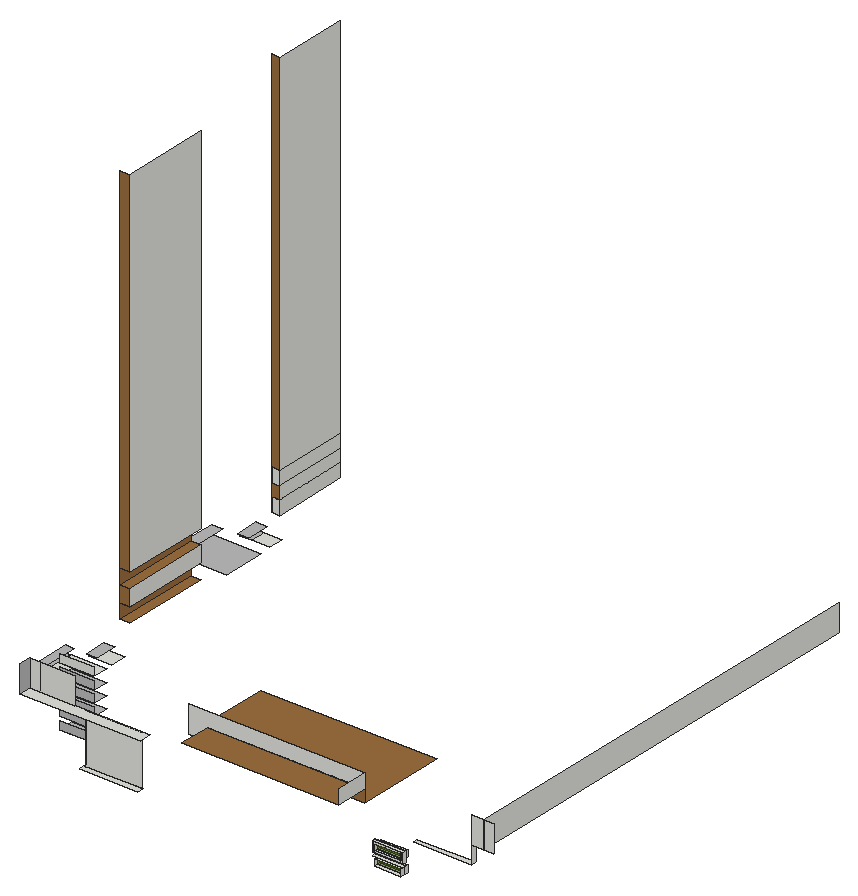
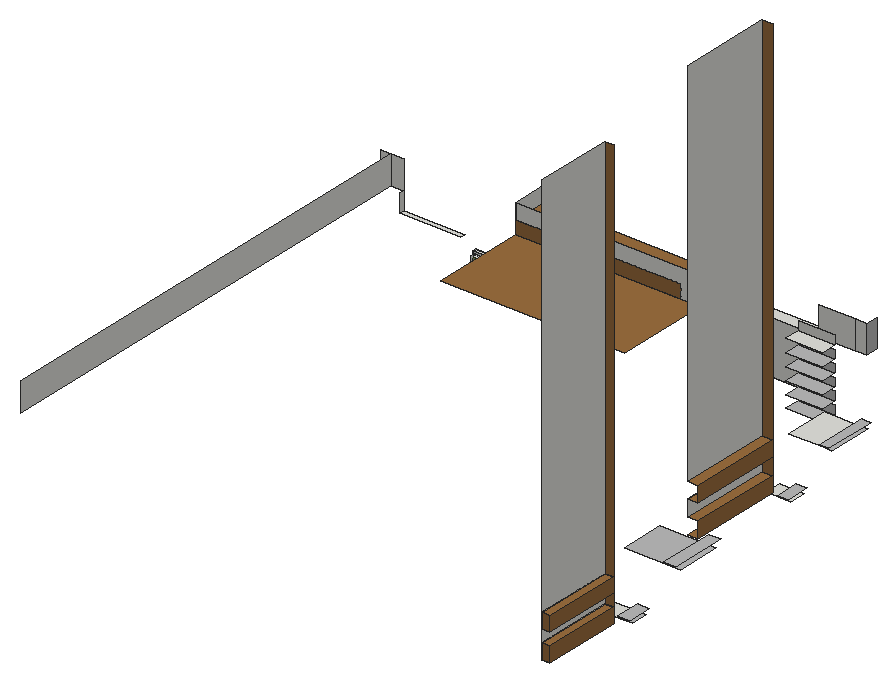
# SketchUp Ruby script. Lengths in inches.
U = 1.inch
M = Sketchup.active_model
def pt(a) = Geom::Point3d.new(a.map { |v| v * U })
def face(e, loops, mat)
  f = e.add_face(loops[0].map { |a| pt(a) })
  loops[1..].each { |l| e.add_face(l.map { |a| pt(a) }).erase! }
  f.material = f.back_material = mat if mat
  f
end
# faces: each face lists its corners as indices into pts; further lists are holes
def faces(e, pts, list, mat = nil) = list.each { |f| face(e, (f[0].is_a?(Array) ? f : [f]).map { |l| l.map { |i| pts[i] } }, mat) }
# xy, xz, yz: faces in a plane at the given z, y or x. An outline is a flat list of corners, or four numbers for a rectangle; further outlines are holes
def ring(l) = l.size == 4 ? [[l[0], l[1]], [l[2], l[1]], [l[2], l[3]], [l[0], l[3]]] : l.each_slice(2).to_a
def flat(e, list, mat, &to3) = list.each { |f| face(e, (f[0].is_a?(Array) ? f : [f]).map { |l| ring(l).map { |u, v| to3.(u, v) } }, mat) }
def xy(e, z, list, mat = nil) = flat(e, list, mat) { |x, y| [x, y, z] }
def xz(e, y, list, mat = nil) = flat(e, list, mat) { |x, z| [x, y, z] }
def yz(e, x, list, mat = nil) = flat(e, list, mat) { |y, z| [x, y, z] }
def lines(e, pts, list) = list.each { |a, b| e.add_line(pt(pts[a]), pt(pts[b])) }
# prism: a flat outline (further loops are holes) pulled along v
def prism(e, loops, v, mat = nil)
  f = face(e, loops, mat); d = Geom::Vector3d.new(v.map { |x| x * U })
  f.pushpull(f.normal.samedirection?(d) ? d.length : -d.length)
end
def box(e, o, s, mat = nil) = prism(e, [[o, [o[0] + s[0], o[1], o[2]], [o[0] + s[0], o[1] + s[1], o[2]], [o[0], o[1] + s[1], o[2]]]], [0, 0, s[2]], mat)
def at(x, y, z, deg = 0) = Geom::Transformation.translation(pt([x, y, z])) * Geom::Transformation.rotation(ORIGIN, Z_AXIS, deg.degrees)
def axes(o, x, y, z) = Geom::Transformation.new([*x, 0, *y, 0, *z, 0, *pt(o).to_a, 1])
def part(name) = M.definitions.add(name)
# library, detail: a bought-in or finely detailed component or shape, given as its bounding box
def library(name, o, s) = part(name).tap { |d| box(d.entities, o, s) }
def detail(e, o, s) = box(e.add_group.entities, o, s)
def put(e, d, t, mat = nil) = e.add_instance(d, t).tap { |i| i.material = mat if mat }
def group(e, t, mat = nil) = e.add_group.tap { |g| g.transformation = t; g.material = mat if mat }.entities
root = M.entities
M.materials.add("Generic").color = [155, 110, 63]
M.materials.add("Generic\#2").color = [186, 186, 186]
M.materials.add("[Translucent Glass Dark Green]").color = [62, 91, 5]
M.materials["[Translucent Glass Dark Green]"].alpha = 0.5
c1 = part("Group\#7")
xy(c1.entities,0,[[0,0,36.1875,3]])
xy(c1.entities,8.75,[[0,0,36.1875,3]])
xz(c1.entities,0,[[0,0,36.1875,8.75]],"[Translucent Glass Dark Green]")
xz(c1.entities,3,[[0,0,36.1875,8.75]],"[Translucent Glass Dark Green]")
yz(c1.entities,0,[[0,0,3,8.75]])
yz(c1.entities,36.1875,[[0,0,3,8.75]])
c2 = part("Group\#1")
xy(c2.entities,0,[[0,0,46.77,20.375]])
xz(c2.entities,0,[[0,0,46.77,11.0625]])
xy(root,304.59,[[170.35,89.25,249.19,97.25]])
xy(root,304.68,[[545.16,120,581.35,124.5],[545.16,124.5,581.35,130.75]])
xy(root,311.95,[[34.5,275.13,65.625,296.69]])
xy(root,313.43,[[545.16,120,581.35,124.5],[545.16,124.5,581.35,130.75]])
xy(root,314.51,[[15.3125,574.26,39.625,595.82]])
xy(root,314.51,[[0,574.26,15.3125,595.82]],"Generic\#2")
xy(root,316.04,[[542.55,120,583.96,124.5]])
xy(root,316.16,[[34.5,270.92,48.5,300.91]],"Generic\#2")
xy(root,319.35,[[0,569.42,15.3125,600.66]],"Generic\#2")
xy(root,320.57,[[542.55,120,583.96,124.5]])
xy(root,323.18,[[545.16,120,581.35,124.5],[545.16,124.5,581.35,130.75]])
xy(root,323.59,[[4.375,621.86,15.3125,724.5]],"Generic")
xy(root,331.93,[[545.16,120,581.35,124.5],[545.16,124.5,581.35,130.75]])
xy(root,334.54,[[542.55,120,583.96,124.5]])
xy(root,334.69,[[35,326.1875,48.5,446.1875]],"Generic")
xy(root,339.6,[[48.5,169.34,93.0625,226.78]])
xy(root,339.6,[[37,169.34,48.5,226.78]],"Generic\#2")
xy(root,342.41,[[0,461.22,72.5625,518.66]],"Generic\#2")
xy(root,342.85,[[4.375,621.86,15.3125,724.5]],"Generic")
xy(root,344.75,[[37,164.2,48.5,231.93]],"Generic\#2")
xy(root,349.35,[[594.67,124.5,673.48,130.75]])
xy(root,349.56,[[0,454.08,15.3125,525.8]],"Generic\#2")
xy(root,354.7,[[35,326.1875,48.5,446.1875]],"Generic")
xy(root,359.01,[[4.375,621.86,15.3125,724.5]],"Generic")
xy(root,372.9375,[[96.41,81.125,259.3125,97.25]])
xy(root,372.9375,[[290.4375,124.5,528.75,246]],"Generic")
xy(root,376.31,[[35,326.1875,48.5,446.1875]],"Generic")
xy(root,378.21,[[4.375,621.86,15.3125,724.5]],"Generic")
xy(root,390.1875,[[315.5625,81.125,528.75,124.5]],"Generic")
xy(root,396.32,[[35,326.1875,48.5,446.1875]],"Generic")
xz(root,97.25,[[172.53,304.59,173.03,372.9375],[173.03,304.59,247.78,372.9375],[247.78,304.59,248.28,372.9375],[96.41,372.9375,110.7,409.46],[110.7,372.9375,157.47,409.46]])
xz(root,120,[[[542.55,320.57,583.96,334.54],[545.16,323.18,581.35,331.93]]])
xz(root,124.5,[[[542.55,320.57,583.96,334.54],[545.16,323.18,581.35,331.93]],[290.4375,372.9375,290.4375,409.875,528.75,409.875,528.75,390.1875,315.5625,390.1875,315.5625,372.9375],[673.48,372.9375,690.4375,409.875],[690.4375,372.9375,703.6875,409.875]])
xz(root,124.5,[[315.5625,372.9375,528.75,390.1875]],"Generic")
xz(root,326.1875,[[35,354.7,48.5,376.31],[35,396.32,48.5,878.88]],"Generic")
xz(root,621.86,[[4.375,323.59,15.3125,342.85],[4.375,359.01,15.3125,378.21]])
xz(root,621.86,[[4.375,342.85,15.3125,359.01],[4.375,378.21,15.3125,879.52]],"Generic")
xz(root,724.5,[[4.375,323.59,15.3125,342.85],[4.375,359.01,15.3125,378.21]],"Generic")
yz(root,4.375,[[621.86,323.59,724.5,342.85],[621.86,359.01,724.5,378.21]],"Generic")
yz(root,15.3125,[[621.86,323.59,724.5,342.85],[621.86,342.85,724.5,359.01],[621.86,359.01,724.5,378.21],[621.86,378.21,724.5,879.52]])
yz(root,35,[[326.1875,334.69,446.1875,354.7],[326.1875,376.31,446.1875,396.32]],"Generic")
yz(root,48.5,[[326.1875,354.7,446.1875,376.31],[326.1875,396.32,446.1875,878.88]])
yz(root,96.41,[[81.125,372.9375,97.25,409.46]],"Generic\#2")
yz(root,528.75,[[81.125,390.1875,124.5,409.875]])
yz(root,542.55,[[120,320.57,124.5,334.54]])
yz(root,545.16,[[120,304.68,124.5,313.43],[124.5,304.68,130.75,313.43],[120,323.18,124.5,331.93],[124.5,323.18,130.75,331.93]])
yz(root,581.35,[[120,304.68,124.5,313.43],[124.5,304.68,130.75,313.43],[120,323.18,124.5,331.93],[124.5,323.18,130.75,331.93]])
yz(root,583.96,[[120,320.57,124.5,334.54]])
yz(root,673.48,[[124.5,349.35,130.75,372.9375]])
yz(root,690.4375,[[124.5,372.9375,724.5,409.875]])
put(root,c1,at(545.16,124.5,304.68))
put(root,c2,at(110.7,130.3125,313),"Generic\#2")
put(root,c1,at(545.16,124.5,323.18))
put(root,c2,at(110.7,130.3125,329.1875),"Generic\#2")
put(root,c2,at(110.7,130.3125,345.375),"Generic\#2")
put(root,c2,at(110.7,130.3125,361.5625),"Generic\#2")
put(root,c2,at(110.7,130.3125,377.75),"Generic\#2")
put(root,c2,at(110.7,130.3125,394.375))
